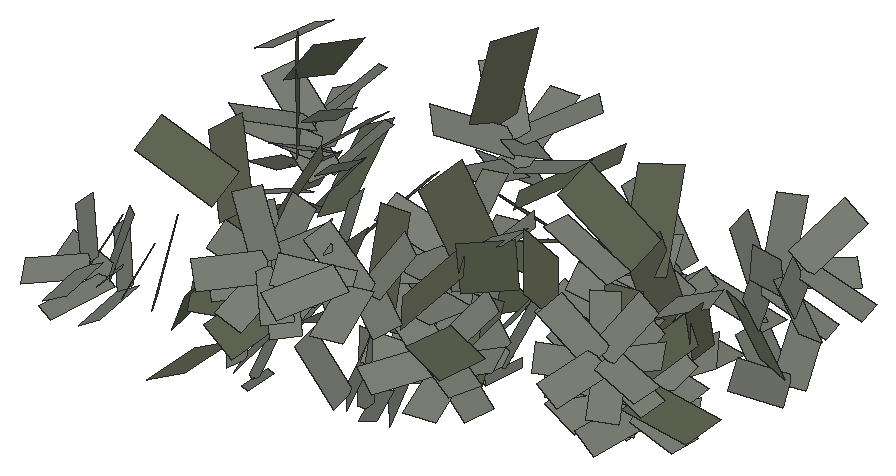
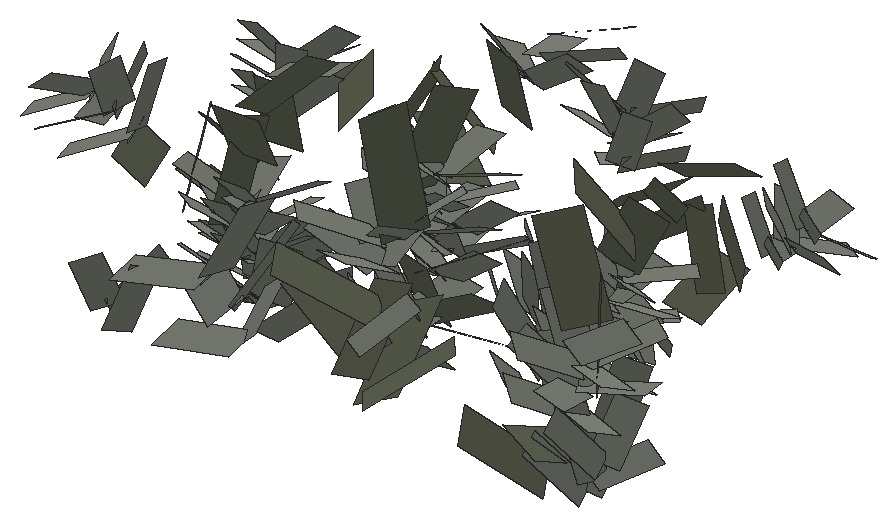
# SketchUp Ruby script. Lengths in inches.
U = 1.inch
M = Sketchup.active_model
def pt(a) = Geom::Point3d.new(a.map { |v| v * U })
def face(e, loops, mat)
  f = e.add_face(loops[0].map { |a| pt(a) })
  loops[1..].each { |l| e.add_face(l.map { |a| pt(a) }).erase! }
  f.material = f.back_material = mat if mat
  f
end
# faces: each face lists its corners as indices into pts; further lists are holes
def faces(e, pts, list, mat = nil) = list.each { |f| face(e, (f[0].is_a?(Array) ? f : [f]).map { |l| l.map { |i| pts[i] } }, mat) }
# xy, xz, yz: faces in a plane at the given z, y or x. An outline is a flat list of corners, or four numbers for a rectangle; further outlines are holes
def ring(l) = l.size == 4 ? [[l[0], l[1]], [l[2], l[1]], [l[2], l[3]], [l[0], l[3]]] : l.each_slice(2).to_a
def flat(e, list, mat, &to3) = list.each { |f| face(e, (f[0].is_a?(Array) ? f : [f]).map { |l| ring(l).map { |u, v| to3.(u, v) } }, mat) }
def xy(e, z, list, mat = nil) = flat(e, list, mat) { |x, y| [x, y, z] }
def xz(e, y, list, mat = nil) = flat(e, list, mat) { |x, z| [x, y, z] }
def yz(e, x, list, mat = nil) = flat(e, list, mat) { |y, z| [x, y, z] }
def lines(e, pts, list) = list.each { |a, b| e.add_line(pt(pts[a]), pt(pts[b])) }
# prism: a flat outline (further loops are holes) pulled along v
def prism(e, loops, v, mat = nil)
  f = face(e, loops, mat); d = Geom::Vector3d.new(v.map { |x| x * U })
  f.pushpull(f.normal.samedirection?(d) ? d.length : -d.length)
end
def box(e, o, s, mat = nil) = prism(e, [[o, [o[0] + s[0], o[1], o[2]], [o[0] + s[0], o[1] + s[1], o[2]], [o[0], o[1] + s[1], o[2]]]], [0, 0, s[2]], mat)
def at(x, y, z, deg = 0) = Geom::Transformation.translation(pt([x, y, z])) * Geom::Transformation.rotation(ORIGIN, Z_AXIS, deg.degrees)
def axes(o, x, y, z) = Geom::Transformation.new([*x, 0, *y, 0, *z, 0, *pt(o).to_a, 1])
def part(name) = M.definitions.add(name)
# library, detail: a bought-in or finely detailed component or shape, given as its bounding box
def library(name, o, s) = part(name).tap { |d| box(d.entities, o, s) }
def detail(e, o, s) = box(e.add_group.entities, o, s)
def put(e, d, t, mat = nil) = e.add_instance(d, t).tap { |i| i.material = mat if mat }
def group(e, t, mat = nil) = e.add_group.tap { |g| g.transformation = t; g.material = mat if mat }.entities
root = M.entities
M.materials.add("viburnumblaasdfas0df1w06d").color = [98, 102, 84]
M.materials.add("viburnumbladsadfasdfad0w122").color = [125, 129, 119]
c1 = part("Component\#315")
p = [[0.25,0,0],[2.05,0.01,0.35],[1.81,4.2,1.66],[0,4.19,1.3125]]
faces(c1.entities,p,[[0,1,2,3]],"viburnumbladsadfasdfad0w122")
c2 = part("viburnumblad2")
put(c2.entities,c1,axes([-19.23,-4.49,-32.18],[83.35428,0,0],[0,79.38502,0],[0,0,83.35428]))
c3 = part("Component\#314")
p = [[0.14,0,0],[2.58,0.05,0.25],[2.44,5.11,2.64],[0,5.05,2.39]]
faces(c3.entities,p,[[0,1,2,3]],"viburnumblaasdfas0df1w06d")
c4 = part("viburnumblad1\#2")
put(c4.entities,c3,axes([-37.25,6.23,19.31],[75.98784,0,0],[0,65.50676,0],[0,0,75.98784]))
put(root,c2,axes([2210.98,245.61,41],[-0.00995,0.00489,0.00397],[-0.00628,-0.00876,-0.0047],[0.00102,-0.00608,0.00892]))
put(root,c2,axes([2194.08,246.49,36.46],[-0.00855,-0.00051,-0.00592],[0.00282,-0.00961,-0.00317],[-0.00532,-0.00402,0.00702]))
put(root,c2,axes([2211.35,247.21,40.45],[-0.01153,-0.00217,-0.00126],[0.00257,-0.00998,-0.00587],[-0.00007,-0.00594,0.00905]))
put(root,c2,axes([2194.73,246.58,35.24],[-0.00848,0.00604,-0.00136],[-0.00422,-0.00741,-0.00622],[-0.00446,-0.0043,0.00739]))
put(root,c2,axes([2204.71,247.03,38.64],[-0.00593,0.00534,0.00783],[-0.0086,-0.00691,-0.00181],[0.00397,-0.00698,0.00778]))
put(root,c2,axes([2193.45,245.78,35.56],[-0.00345,0.00905,0.004],[-0.00908,-0.00113,-0.00507],[-0.00385,-0.00506,0.00725]))
put(root,c2,axes([2195.31,247.78,34.96],[-0.00729,-0.00007,-0.00611],[0.00282,-0.00961,-0.00317],[-0.00621,-0.00405,0.00634]))
put(root,c2,axes([2210.35,246.29,39.8],[-0.00254,0.00908,0.00688],[-0.01141,-0.00302,-0.00024],[0.00165,-0.00679,0.00837]))
put(root,c2,axes([2194.26,247.87,35.79],[-0.0036,-0.00676,-0.00701],[0.00718,-0.00608,0.00197],[-0.00593,-0.00439,0.00637]))
put(root,c2,axes([2205.21,248.04,39.49],[-0.00902,-0.00601,-0.00274],[0.00624,-0.00625,-0.00686],[0.00215,-0.00706,0.0084]))
put(root,c2,axes([2193.1,247.39,36.44],[0.00345,-0.00905,-0.004],[0.00788,-0.00012,0.00668],[-0.00594,-0.00519,0.00581]))
put(root,c2,axes([2204.74,248.61,38.12],[-0.01058,-0.00047,0.0036],[-0.00191,-0.00936,-0.00683],[0.00314,-0.00674,0.00835]))
put(root,c2,axes([2210.85,248.58,39.97],[-0.00572,-0.00664,-0.00612],[0.0099,-0.00571,-0.00294],[-0.00165,-0.00728,0.00803]))
put(root,c2,axes([2194.49,248.56,34.85],[0.0036,-0.00945,-0.00418],[0.00709,-0.00011,0.00601],[-0.00594,-0.00519,0.00581]))
put(root,c2,axes([2193.57,246.69,34.57],[0.0036,0.00676,0.00701],[-0.00902,0.00536,-0.00055],[-0.00386,-0.00586,0.0067]))
put(root,c2,axes([2192.47,246.68,35.54],[0.00855,0.00051,0.00592],[-0.00403,0.00835,0.00477],[-0.00448,-0.00623,0.00604]))
put(root,c2,axes([2203.74,247.87,37.72],[0.00218,0.00802,0.00747],[-0.00931,-0.0013,0.00412],[0.00416,-0.00766,0.007]))
put(root,c2,axes([2203.44,247.14,39.25],[0.00902,0.00601,0.00274],[-0.00554,0.00435,0.00868],[0.0036,-0.00837,0.00649]))
put(root,c2,axes([2203.78,248.93,36.85],[-0.0062,0.00558,0.00817],[-0.00774,-0.00622,-0.00163],[0.00397,-0.00698,0.00778]))
put(root,c2,axes([2193.28,247.72,35.06],[0.00848,-0.00604,0.00136],[0.00312,0.00638,0.00815],[-0.00533,-0.00595,0.00568]))
put(root,c2,axes([2204.16,249.98,37.74],[-0.00866,-0.00577,-0.00263],[0.00674,-0.00675,-0.0074],[0.00215,-0.00706,0.0084]))
put(root,c4,axes([2199,251.1875,31.14],[-0.01085,-0.00246,-0.00558],[0.00478,-0.01321,-0.00344],[-0.00438,-0.00417,0.00964]))
put(root,c2,axes([2209.78,247.375,38.95],[0.00611,0.00764,0.00552],[-0.01063,0.0043,0.00535],[0.00146,-0.00765,0.00773]))
put(root,c2,axes([2203.94,248.15,40.1],[0.00593,-0.00534,-0.00783],[0.00931,0.00502,0.00364],[0.00177,-0.00845,0.00711]))
put(root,c4,axes([2203.52,251.18,35.08],[-0.00973,0.00003,0.00746],[-0.00524,-0.01136,-0.00678],[0.00594,-0.00739,0.00778]))
put(root,c2,axes([2204.17,249.26,39.05],[-0.00218,-0.00802,-0.00747],[0.01085,-0.00048,-0.00266],[0.00158,-0.00777,0.00788]))
put(root,c2,axes([2209.59,248.52,39.87],[0.01038,-0.0051,-0.00415],[0.00571,0.00633,0.00604],[-0.00053,-0.00802,0.00751]))
put(root,c2,axes([2193.96,247.78,33.93],[0.00821,0.00049,0.00568],[-0.00435,0.00902,0.00515],[-0.00448,-0.00623,0.00604]))
put(root,c4,axes([2196.98,251,32.46],[-0.00104,-0.01037,-0.00489],[0.01073,-0.00422,0.00645],[-0.0067,-0.00317,0.00766]))
put(root,c2,axes([2202.91,248.6,38.84],[0.01058,0.00047,-0.0036],[0.00255,0.00709,0.00842],[0.00261,-0.00869,0.00653]))
put(root,c4,axes([2195.3,249.85,32.91],[0.00672,-0.00928,0.00091],[0.00601,0.00561,0.01016],[-0.00772,-0.00461,0.00599]))
put(root,c2,axes([2202.7,248.93,37.39],[0.0079,0.00633,0.00186],[-0.00554,0.00435,0.00868],[0.00455,-0.00767,0.00675]))
put(root,c4,axes([2202.2,251.8,33.3125],[-0.0017,0.006,0.01056],[-0.01273,-0.00619,0.00147],[0.00521,-0.00927,0.00611]))
put(root,c2,axes([2223.12,252.09,37.56],[-0.00968,0.00131,0.00494],[-0.00342,-0.0096,-0.00398],[0.00374,-0.00505,0.00789]))
put(root,c4,axes([2209.18,249.93,37.5],[0.01273,-0.00184,0.00122],[0.00029,0.0105,0.01027],[-0.0024,-0.00896,0.00784]))
put(root,c4,axes([2211.03,253.68,35.06],[-0.00662,-0.01127,-0.00498],[0.01432,-0.00702,-0.0031],[-0.00011,-0.00548,0.01154]))
put(root,c4,axes([2198.26,251.09,39.05],[0.0023,0.0101,0.00657],[-0.0138,0.00343,-0.00044],[-0.0019,-0.0063,0.01035]))
put(root,c2,axes([2199.6,253.16,29.28],[-0.00404,-0.00727,-0.00631],[0.00772,-0.00559,0.00142],[-0.00472,-0.00433,0.00722]))
put(root,c2,axes([2222.91,253.6,37.07],[-0.00956,-0.00538,0.00002],[0.00454,-0.00801,-0.00608],[0.00277,-0.00525,0.00814]))
put(root,c4,axes([2209.58,252.1,36.74],[0.00746,-0.00961,-0.00443],[0.01187,0.00604,0.00656],[-0.00274,-0.0068,0.00947]))
put(root,c2,axes([2222.24,252.5,36.54],[-0.00413,0.00723,0.00696],[-0.00909,-0.00609,0.00092],[0.00444,-0.00548,0.00729]))
put(root,c2,axes([2211.08,253.23,32.95],[-0.00995,0.00489,0.00397],[-0.00607,-0.00954,-0.00338],[0.0019,-0.00477,0.00949]))
put(root,c2,axes([2222.8125,253.1,38.42],[-0.00385,-0.00891,-0.00491],[0.01001,-0.00205,-0.00401],[0.00209,-0.00597,0.00789]))
put(root,c2,axes([2198.58,252.66,30.09],[0.00345,-0.00905,-0.004],[0.00865,0.00062,0.00578],[-0.00475,-0.00515,0.0067]))
put(root,c2,axes([2221.84,251.57,37.71],[0.00385,0.00891,0.00491],[-0.00921,0.00054,0.0058],[0.00445,-0.00629,0.00669]))
put(root,c2,axes([2205.17,252.5,30.47],[0.00814,-0.00715,-0.0046],[0.00716,0.00216,0.00888],[-0.00455,-0.00881,0.00477]))
put(root,c2,axes([2206.23,253.59,30.01],[0.00034,-0.00733,-0.00907],[0.00978,-0.00348,0.00299],[-0.00497,-0.00808,0.00546]))
put(root,c2,axes([2201.07,254.11,33.14],[-0.0105,0.00104,-0.00371],[-0.00071,-0.0111,-0.00111],[-0.00379,-0.00081,0.01049]))
put(root,c2,axes([2200.22,253.1,34.15],[-0.00725,0.00846,-0.00094],[-0.008,-0.0072,-0.00303],[-0.00289,-0.00129,0.01072]))
put(root,c2,axes([2204.97,251.64,29.28],[0.00766,0.00322,0.00823],[-0.00853,0.00606,0.00527],[-0.00262,-0.00929,0.00521]))
put(root,c2,axes([2200.47,254.44,34.53],[-0.00759,-0.00699,-0.00431],[0.00673,-0.00866,0.00218],[-0.0047,-0.00111,0.01008]))
put(root,c2,axes([2211.33,254.75,32.21],[-0.01146,-0.00283,-0.00038],[0.00275,-0.01049,-0.00491],[0.00082,-0.00467,0.00968]))
put(root,c2,axes([2211,254.51,33.7],[-0.00626,-0.00889,-0.00451],[0.01001,-0.00557,-0.00285],[-0.00007,-0.00526,0.00943]))
put(root,c2,axes([2197.88,251.875,29.29],[0.00916,0.00124,0.00492],[-0.00387,0.00837,0.00487],[-0.00322,-0.0061,0.00681]))
put(root,c2,axes([2201.2,253.98,31.65],[-0.00696,0.00812,-0.0009],[-0.00864,-0.00777,-0.00327],[-0.00289,-0.00129,0.01072]))
put(root,c4,axes([2200.31,253.49,32.35],[0.01074,0.00549,0.00552],[-0.0086,0.00502,0.01173],[0.00238,-0.01127,0.00657]))
put(root,c2,axes([2198.55,252.93,28.67],[0.00892,-0.00552,0.00065],[0.00374,0.00694,0.00752],[-0.00413,-0.00589,0.00653]))
put(root,c2,axes([2221.53,252.59,38.57],[0.00968,-0.00131,-0.00494],[0.00422,0.00809,0.00577],[0.0028,-0.00722,0.00669]))
put(root,c2,axes([2222.01,254.66,36.73],[-0.00372,-0.00756,-0.00527],[0.01001,-0.00205,-0.00401],[0.00166,-0.0069,0.00731]))
put(root,c2,axes([2210.34,253.72,31.72],[-0.00261,0.00974,0.006],[-0.01123,-0.00353,0.00072],[0.00254,-0.00551,0.00899]))
put(root,c2,axes([2205.4,253.14,29.01],[0.01118,-0.00278,0.00257],[-0.00082,0.00655,0.0102],[-0.00357,-0.00931,0.00467]))
put(root,c2,axes([2221.32,253.28,35.86],[0.00369,0.00856,0.00471],[-0.00994,0.00059,0.00626],[0.00445,-0.00629,0.00669]))
put(root,c2,axes([2221.53,253.81,37.75],[0.00413,-0.00723,-0.00696],[0.00908,0.00421,0.0008],[0.0021,-0.00679,0.00729]))
put(root,c4,axes([2197.78,252.36,37.22],[0.01004,0.00303,0.00636],[-0.00636,0.01197,0.00433],[-0.00443,-0.0059,0.0098]))
put(root,c2,axes([2221.18,252.74,37.13],[0.00956,0.00538,-0.00002],[-0.00388,0.00674,0.0082],[0.00377,-0.00701,0.00644]))
put(root,c2,axes([2206.29,254.55,29.09],[0.0085,-0.00746,-0.0048],[0.00645,0.00195,0.00799],[-0.00455,-0.00881,0.00477]))
put(root,c2,axes([2209.59,253.09,33.03],[0.00626,0.00889,0.00451],[-0.00973,0.00413,0.00504],[0.00235,-0.00645,0.00846]))
put(root,c2,axes([2200.15,253.41,32.62],[0.00024,0.01092,0.00238],[-0.01143,0.00081,-0.00255],[-0.00254,-0.00227,0.01065]))
put(root,c2,axes([2200.3,255.32,33.1],[-0.00024,-0.01092,-0.00238],[0.01005,-0.00131,0.00499],[-0.0051,-0.00202,0.00975]))
put(root,c2,axes([2210.73,256.02,31.61],[-0.00572,-0.00761,-0.00506],[0.01001,-0.00557,-0.00285],[-0.00075,-0.00619,0.00889]))
put(root,c4,axes([2213.08,256.98,37.12],[-0.00612,0.00474,0.0114],[-0.00511,-0.01476,0.0034],[0.01154,-0.00234,0.00716]))
put(root,c2,axes([2210.47,256.54,38.125],[-0.01249,0.00076,-0.00112],[-0.00058,-0.01239,-0.00197],[-0.00123,-0.0019,0.01236]))
put(root,c2,axes([2209.92,255.46,32.74],[0.00261,-0.00974,-0.006],[0.01057,0.00192,0.00135],[-0.00026,-0.0062,0.0089]))
put(root,c4,axes([2214.61,257.77,39.02],[-0.00769,-0.00672,0.00925],[0.00492,-0.01396,-0.00605],[0.01062,-0.00006,0.00878]))
put(root,c2,axes([2220.91,254.23,36.77],[0.01011,-0.00136,-0.00516],[0.0038,0.00729,0.00519],[0.0028,-0.00722,0.00669]))
put(root,c2,axes([2209.52,254.36,33.79],[0.00995,-0.00489,-0.00397],[0.00635,0.0081,0.00558],[0.00038,-0.00694,0.0084]))
put(root,c4,axes([2198.54,254.38,35.57],[0.00884,-0.00966,0.00214],[0.00883,0.00982,0.0079],[-0.00632,-0.00331,0.01118]))
put(root,c2,axes([2198.92,253.47,33.74],[0.00759,0.00699,0.00431],[-0.00767,0.00813,0.00032],[-0.00293,-0.00317,0.01031]))
put(root,c2,axes([2200.8125,257.29,32.66],[-0.0119,0.00385,-0.00772],[-0.00199,-0.01402,-0.00394],[-0.0084,-0.00214,0.01187]))
put(root,c2,axes([2199.17,254.8,34.11],[0.00725,-0.00846,0.00094],[0.00707,0.00667,0.00553],[-0.00474,-0.00299,0.00967]))
put(root,c2,axes([2210.54,257.68,35.17],[-0.01199,0.00073,-0.00108],[-0.00063,-0.01339,-0.00213],[-0.00123,-0.0019,0.01236]))
put(root,c2,axes([2210.17,256.53,36.4],[-0.00853,0.00907,0.00165],[-0.00968,-0.00877,-0.00184],[-0.00017,-0.0024,0.01233]))
put(root,c2,axes([2209.66,254.64,30.78],[0.00601,0.00853,0.00433],[-0.01051,0.00446,0.00545],[0.00235,-0.00645,0.00846]))
put(root,c2,axes([2199.24,254.34,32.46],[0.0105,-0.00104,0.00371],[-0.00021,0.00971,0.00332],[-0.00385,-0.00347,0.00991]))
put(root,c2,axes([2210.34,257.88,36.82],[-0.00913,-0.008,-0.00324],[0.00831,-0.00942,-0.00017],[-0.00232,-0.00227,0.01214]))
put(root,c2,axes([2199.86,254.22,31.24],[0.00793,0.00729,0.0045],[-0.0069,0.00732,0.00029],[-0.00293,-0.00317,0.01031]))
put(root,c2,axes([2199.99,255.36,31.625],[0.0071,-0.00744,-0.0001],[0.00707,0.00667,0.00553],[-0.00393,-0.00389,0.00972]))
put(root,c2,axes([2209.28,254.36,32.1875],[0.01146,0.00283,0.00038],[-0.00257,0.0094,0.00741],[0.00146,-0.00704,0.00821]))
put(root,c4,axes([2219.86,255.35,34.68],[0.0118,0.00221,-0.00034],[-0.00169,0.00933,0.00984],[0.00149,-0.00861,0.00716]))
put(root,c4,axes([2210.24,257.55,31.83],[-0.0066,0.01089,0.00527],[-0.0139,-0.00777,-0.00135],[0.00164,-0.00514,0.01268]))
put(root,c2,axes([2201.65,258.88,31.42],[-0.00909,-0.00693,-0.00924],[0.00664,-0.01276,0.00304],[-0.00946,-0.0023,0.01102]))
put(root,c2,axes([2209.15,255.74,37.76],[0.00042,0.01207,0.00346],[-0.01255,0.00034,0.00035],[0.00024,-0.00347,0.01207]))
put(root,c2,axes([2209.46,255.89,31.57],[0.01038,-0.0051,-0.00415],[0.00572,0.00729,0.00502],[0.00038,-0.00694,0.0084]))
put(root,c4,axes([2210.23,256.6875,36.08],[0.00411,0.01355,0.00465],[-0.01078,-0.00135,0.01345],[0.01091,-0.00609,0.00813]))
put(root,c2,axes([2216.09,257.6875,42.04],[-0.00224,-0.01174,-0.0016],[0.0107,-0.00091,-0.00829],[0.00736,-0.00274,0.0098]))
put(root,c2,axes([2209.61,257.84,38.4],[-0.00042,-0.01207,-0.00346],[0.01224,-0.00117,0.00258],[-0.0028,-0.00328,0.0118]))
put(root,c2,axes([2209.79,259.3,31.41],[-0.01244,-0.00019,-0.00567],[0.00199,-0.01294,-0.00394],[-0.00531,-0.00441,0.0118]))
put(root,c2,axes([2220,258.82,30.4],[-0.00968,0.00131,0.00494],[-0.00285,-0.01022,-0.00281],[0.00419,-0.00363,0.00837]))
put(root,c2,axes([2200.04,258.98,32.65],[-0.00095,-0.01366,-0.00535],[0.01077,-0.00429,0.00904],[-0.00996,-0.00334,0.01028]))
put(root,c2,axes([2209.29,256.75,34.8125],[0.00044,0.0126,0.00361],[-0.0113,0.00031,0.00032],[0.00024,-0.00347,0.01207]))
put(root,c4,axes([2220.07,259.2,32.36],[-0.00299,-0.01191,-0.00429],[0.01424,-0.00187,-0.0047],[0.00288,-0.00486,0.01046]))
put(root,c4,axes([2219.47,257.38,34.02],[0.00886,-0.00621,-0.00526],[0.00932,0.00889,0.00498],[0.00073,-0.00681,0.00878]))
put(root,c4,axes([2208.83,256.94,29.08],[0.01287,-0.00107,0.00071],[0.00034,0.01171,0.00907],[-0.00141,-0.0079,0.00892]))
put(root,c2,axes([2199.51,256.69,31.47],[0.00095,0.01366,0.00535],[-0.01286,0.00336,-0.00628],[-0.00706,-0.00428,0.01216]))
put(root,c2,axes([2208.7,256.52,36.22],[0.00913,0.008,0.00324],[-0.00792,0.00789,0.00285],[-0.00024,-0.00448,0.01173]))
put(root,c2,axes([2219.07,259.03,29.36],[-0.00449,0.00779,0.00619],[-0.00867,-0.00648,0.00177],[0.0049,-0.00408,0.00781]))
put(root,c2,axes([2218.16,260.82,31.47],[-0.01366,0.00095,0.00535],[-0.00336,-0.01286,-0.00628],[0.00428,-0.00706,0.01216]))
put(root,c2,axes([2208.76,258.21,36.74],[0.00853,-0.00907,-0.00165],[0.009,0.0076,0.00473],[-0.00239,-0.00435,0.01154]))
put(root,c2,axes([2208.29,257.04,38.03],[0.01249,-0.00076,0.00112],[0.00026,0.01157,0.0049],[-0.00133,-0.00485,0.01151]))
put(root,c2,axes([2209.91,260.96,30.23],[-0.00694,-0.00883,-0.00779],[0.00996,-0.00923,0.0016],[-0.00629,-0.00487,0.01112]))
put(root,c4,axes([2209.16,257.96,29.54],[0.0051,0.011,0.00655],[-0.01483,0.00551,0.0023],[-0.00067,-0.00681,0.01196]))
put(root,c2,axes([2219.64,259.92,31.15],[-0.00334,-0.0097,-0.00381],[0.01007,-0.00189,-0.00393],[0.0026,-0.00465,0.00851]))
put(root,c2,axes([2218.76,258.25,30.63],[0.00334,0.0097,0.00381],[-0.00915,0.00071,0.00588],[0.00496,-0.00497,0.00731]))
put(root,c2,axes([2208.7,258.39,30.4375],[-0.00263,0.0123,0.00535],[-0.01296,-0.00091,-0.00426],[-0.00348,-0.00589,0.01184]))
put(root,c4,axes([2218.99,259.29,38.87],[0.00217,0.0115,0.00524],[-0.01369,-0.00006,0.0058],[0.00451,-0.00566,0.01058]))
put(root,c2,axes([2208.62,260.56,31.55],[0.00263,-0.0123,-0.00535],[0.01173,-0.00054,0.007],[-0.00651,-0.00594,0.01045]))
put(root,c2,axes([2219.08,261.55,35.37],[-0.01126,-0.00309,0.00036],[0.00297,-0.01108,-0.00222],[0.00093,-0.00205,0.01147]))
put(root,c2,axes([2208.49,257.8,35.125],[0.01156,-0.00022,-0.00012],[0.00026,0.01157,0.0049],[0.00003,-0.0049,0.01157]))
put(root,c2,axes([2195.63,261.61,29.54],[-0.00877,-0.00751,-0.00615],[0.00336,-0.01013,0.00757],[-0.0091,0.00349,0.00872]))
put(root,c2,axes([2200.17,259.63,30.53],[0.00774,-0.01238,0.00167],[0.00805,0.00648,0.01066],[-0.00962,-0.00465,0.01009]))
put(root,c2,axes([2200.05,257.71,29.75],[0.00909,0.00693,0.00924],[-0.00802,0.01085,-0.00026],[-0.00757,-0.00532,0.01142]))
put(root,c2,axes([2218.625,261.46,33.81],[-0.00997,0.00542,0.0028],[-0.00605,-0.01063,-0.00096],[0.002,-0.00216,0.01131]))
put(root,c2,axes([2198.75,258.38,31.47],[0.0119,-0.00385,0.00772],[-0.0001,0.01309,0.00669],[-0.00863,-0.00547,0.01057]))
put(root,c2,axes([2218.09,259.64,28.61],[0.0032,0.00932,0.00366],[-0.00988,0.00076,0.00635],[0.00496,-0.00497,0.00731]))
put(root,c2,axes([2218.46,262.58,32.67],[-0.01081,-0.00296,0.00035],[0.0032,-0.01197,-0.0024],[0.00093,-0.00205,0.01147]))
put(root,c2,axes([2217.14,261.36,29.75],[-0.00693,0.00909,0.00924],[-0.01085,-0.00802,-0.00026],[0.00532,-0.00757,0.01142]))
put(root,c4,axes([2217.85,262.37,29.62],[-0.0084,0.0076,0.00599],[-0.00998,-0.01102,-0.00002],[0.00443,-0.00403,0.01133]))
put(root,c2,axes([2218.13,260.45,35.14],[-0.00283,0.01075,0.0036],[-0.01102,-0.00348,0.00171],[0.00265,-0.00298,0.01098]))
put(root,c2,axes([2218.31,260.43,30.42],[0.00449,-0.00779,-0.00619],[0.00881,0.00487,0.00016],[0.00266,-0.00553,0.00801]))
put(root,c2,axes([2218.4,259.35,31.39],[0.00968,-0.00131,-0.00494],[0.00378,0.00904,0.00475],[0.00337,-0.00599,0.00744]))
put(root,c2,axes([2216.47,260.05,31.47],[0.00385,0.0119,0.00772],[-0.01309,-0.0001,0.00669],[0.00547,-0.00863,0.01057]))
put(root,c4,axes([2221.12,262.73,34.17],[-0.00543,0.00233,0.01137],[0.00034,-0.01453,0.00314],[0.0116,0.00141,0.00526]))
put(root,c2,axes([2218.01,259.28,29.9375],[0.0092,0.00594,-0.0008],[-0.00419,0.00749,0.00747],[0.00433,-0.00576,0.00715]))
put(root,c2,axes([2217.5625,262.12,32.66],[-0.00385,-0.0119,-0.00772],[0.01402,-0.00199,-0.00394],[0.00214,-0.0084,0.01187]))
put(root,c2,axes([2208.67,259.45,28.82],[0.00694,0.00883,0.00779],[-0.01027,0.00714,0.00105],[-0.0037,-0.00696,0.01117]))
put(root,c2,axes([2200.69,259.26,28.67],[0.01174,-0.00298,0.00601],[-0.0001,0.01309,0.00669],[-0.00729,-0.00586,0.01134]))
put(root,c2,axes([2218.42,262.6875,34.23],[-0.00596,-0.00978,-0.00229],[0.01005,-0.00579,-0.00143],[0.00006,-0.0027,0.01137]))
put(root,c2,axes([2207.53,259.64,30.58],[0.01244,0.00019,0.00567],[-0.00322,0.01148,0.00668],[-0.00467,-0.00741,0.01049]))
put(root,c4,axes([2218.59,261.61,33.51],[0.00008,0.01316,0.00435],[-0.00745,-0.00443,0.01354],[0.01228,-0.00208,0.00607]))
put(root,c2,axes([2217.6,261.38,32.45],[-0.00295,0.01122,0.00376],[-0.00992,-0.00313,0.00154],[0.00265,-0.00298,0.01098]))
put(root,c2,axes([2224.84,263.32,37.51],[-0.00724,-0.00234,0.00954],[0.00229,-0.01023,-0.00078],[0.00905,0.00148,0.00724]))
put(root,c2,axes([2227.21,263.54,39.16],[-0.00693,-0.00224,0.00913],[0.00254,-0.01137,-0.00086],[0.00905,0.00148,0.00724]))
put(root,c2,axes([2208.29,261.17,29.61],[0.01065,-0.00857,0.00023],[0.00633,0.00812,0.0092],[-0.00584,-0.00699,0.01019]))
put(root,c2,axes([2217.64,260.67,29.41],[0.01011,-0.00136,-0.00516],[0.0034,0.00814,0.00428],[0.00337,-0.00599,0.00744]))
put(root,c4,axes([2222.4375,263.88,35.79],[-0.00364,-0.00823,0.00913],[0.00776,-0.0108,-0.00665],[0.01031,0.00314,0.00694]))
put(root,c2,axes([2225.9,262.9,38.375],[-0.00591,0.00652,0.00769],[-0.00251,-0.00882,0.00556],[0.0097,0.00126,0.00639]))
put(root,c2,axes([2217.97,262.4375,35.76],[0.00283,-0.01075,-0.0036],[0.01134,0.00265,0.001],[-0.0001,-0.00373,0.01107]))
put(root,c2,axes([2217.33,261,33.8],[0.00596,0.00978,0.00229],[-0.00894,0.00456,0.00379],[0.00249,-0.00402,0.01069]))
put(root,c2,axes([2215.59,262,28.67],[0.00298,0.01174,0.00601],[-0.01309,-0.0001,0.00669],[0.00586,-0.00729,0.01134]))
put(root,c2,axes([2225.68,264.23,38.67],[-0.0039,-0.00969,0.00523],[0.00734,-0.00679,-0.00711],[0.00851,0.00087,0.00796]))
put(root,c4,axes([2217.27,260.72,37.12],[0.01321,0.00417,0.00061],[-0.00463,0.0136,0.00723],[0.00136,-0.00611,0.01237]))
put(root,c2,axes([2215.875,261.35,32.65],[0.01366,-0.00095,-0.00535],[0.00429,0.01077,0.00904],[0.00334,-0.00996,0.01028]))
put(root,c2,axes([2224.42,262.37,38.22],[-0.0023,0.01045,0.001],[-0.00575,-0.00222,0.00993],[0.00986,0.00159,0.00606]))
put(root,c2,axes([2215.22,261.47,30.53],[0.01238,0.00774,0.00167],[-0.00648,0.00805,0.01066],[0.00465,-0.00962,0.01009]))
put(root,c2,axes([2217.02,261.34,35.54],[0.01126,0.00309,-0.00036],[-0.00265,0.01026,0.00493],[0.00162,-0.00467,0.01059]))
put(root,c2,axes([2215.97,262.96,31.42],[0.00693,-0.00909,-0.00924],[0.01276,0.00664,0.00304],[0.0023,-0.00946,0.01102]))
put(root,c2,axes([2194.78,265.26,35.14],[-0.01197,-0.00238,-0.00293],[0.00194,-0.01232,0.00219],[-0.00304,0.00182,0.01144]))
put(root,c2,axes([2193.98,264.39,36.52],[-0.01008,0.00703,-0.00261],[-0.00714,-0.01028,-0.00011],[-0.00193,0.00159,0.01172]))
put(root,c4,axes([2206.62,266.62,29.26],[-0.01489,-0.00148,0.00524],[0.00198,-0.01828,0.00047],[0.00517,0.00094,0.01496]))
put(root,c2,axes([2207,265.66,37.82],[-0.01229,-0.00021,0.00042],[0.00023,-0.01336,0.00026],[0.00045,0.00027,0.01335]))
put(root,c2,axes([2216.93,262.5,34.34],[0.00997,-0.00542,-0.0028],[0.00614,0.00939,0.00366],[0.00055,-0.00455,0.01075]))
put(root,c2,axes([2206.8,264.61,39.26],[-0.00935,0.00927,0.0023],[-0.00914,-0.00973,0.00201],[0.00303,-0.00016,0.01302]))
put(root,c2,axes([2216.63,262.0625,32.86],[0.01014,0.00329,-0.00138],[-0.00265,0.01026,0.00493],[0.00283,-0.00431,0.01049]))
put(root,c2,axes([2224.1,264.25,38.4],[0.00136,-0.01101,-0.00167],[0.00866,0.00241,-0.00886],[0.00838,-0.00019,0.00814]))
put(root,c4,axes([2193.41,266.07,38.15],[-0.00759,-0.01277,-0.00082],[0.01374,-0.0085,0.0061],[-0.0047,0.00228,0.01321]))
put(root,c2,axes([2226.56,264.5625,40],[0.00142,-0.01147,-0.00174],[0.00801,0.00224,-0.0082],[0.00838,-0.00019,0.00814]))
put(root,c2,axes([2193.96,265.97,36.49],[-0.00685,-0.0104,-0.00154],[0.00967,-0.00694,0.00401],[-0.00399,0.00118,0.01121]))
put(root,c2,axes([2194.63,266.02,33.71],[-0.00587,-0.00963,-0.00252],[0.00967,-0.00694,0.00401],[-0.00471,0.00005,0.01098]))
put(root,c2,axes([2224.95,262.59,39.68],[0.0039,0.00969,-0.00523],[-0.00478,0.00655,0.00858],[0.00995,-0.00072,0.00609]))
put(root,c2,axes([2206.8,266.49,39.42],[-0.00935,-0.00954,0.00039],[0.00874,-0.00859,-0.00062],[0.00075,-0.0002,0.01334]))
put(root,c2,axes([2217.18,266.92,33.6],[-0.01234,0.00028,0.00961],[0.00075,-0.01555,0.00142],[0.00958,0.00158,0.01226]))
put(root,c4,axes([2192.77,264.91,34.28],[0.0095,-0.01111,0.00288],[0.00361,0.00703,0.01484],[-0.01096,-0.00785,0.00554]))
put(root,c2,axes([2193.72,264.07,34.9],[-0.00228,0.01232,-0.00076],[-0.01222,-0.00233,-0.0015],[-0.0013,0.00061,0.01189]))
put(root,c2,axes([2214.99,267.08,30.57],[-0.01223,0.0001,0.00757],[0.00075,-0.01555,0.00142],[0.00819,0.0016,0.01322]))
put(root,c2,axes([2215.65,266,32.24],[-0.00842,0.01125,0.00685],[-0.00786,-0.01092,0.00827],[0.01063,0.001,0.01143]))
put(root,c2,axes([2192.64,266.87,30.28],[-0.00935,-0.0054,-0.00582],[0.00328,-0.00946,0.00316],[-0.00651,0.0014,0.00804]))
put(root,c4,axes([2205.18,266.3125,39.27],[-0.00382,-0.01538,-0.00062],[0.0121,-0.00355,0.01339],[-0.01131,0.00237,0.01086]))
put(root,c2,axes([2191.99,266.45,31.29],[-0.00946,0.00383,-0.00571],[-0.0036,-0.01015,-0.00104],[-0.00558,0.00147,0.00861]))
put(root,c2,axes([2191.2,267.12,32.39],[-0.00896,-0.00518,-0.00557],[0.00365,-0.01051,0.00351],[-0.00651,0.0014,0.00804]))
put(root,c2,axes([2224.91,264.09,39.73],[0.00591,-0.00652,-0.00769],[0.005,0.00963,-0.00433],[0.00875,-0.0011,0.00766]))
put(root,c2,axes([2223.21,266.28,29.28],[-0.00322,0.00766,0.00823],[-0.00606,-0.00853,0.00527],[0.00929,-0.00262,0.00521]))
put(root,c2,axes([2225.94,263.5,40.82],[0.00693,0.00224,-0.00913],[-0.00028,0.01139,0.00259],[0.0094,-0.00132,0.00681]))
put(root,c2,axes([2193.37,266.25,34.74],[0.00228,-0.01232,0.00076],[0.0106,0.00221,0.00397],[-0.00422,0.00003,0.01117]))
put(root,c2,axes([2206.11,266.78,37.96],[0,-0.01388,-0.00141],[0.01203,0.00003,-0.00025],[0.00028,-0.00135,0.01329]))
put(root,c2,axes([2215.68,268.21,32.22],[-0.00902,-0.01086,0.00673],[0.00875,-0.01029,-0.00487],[0.0085,0.00104,0.01308]))
put(root,c4,axes([2206.01,267.69,32.27],[-0.00484,-0.01365,0.00231],[0.016,-0.00575,-0.00049],[0.00117,0.00203,0.01447]))
put(root,c2,axes([2192.44,264.36,36.14],[0.00685,0.0104,0.00154],[-0.01034,0.00702,-0.00117],[-0.00153,-0.00054,0.01185]))
put(root,c2,axes([2193.51,264.34,33.32],[0.00658,0.00998,0.00148],[-0.01117,0.00758,-0.00127],[-0.00153,-0.00054,0.01185]))
put(root,c2,axes([2191.38,267.65,30.96],[-0.00321,-0.01115,-0.00217],[0.00909,-0.00398,0.00703],[-0.00713,0.00058,0.00765]))
put(root,c4,axes([2206.05,267.24,30.4],[-0.00859,0.01076,0.00042],[-0.01222,-0.00981,0.0027],[0.00229,0.0015,0.01233]))
put(root,c4,axes([2206.31,268.875,32.21],[-0.01366,0.00026,0.00163],[0.00037,-0.01516,0.00432],[0.00177,0.00434,0.01188]))
put(root,c2,axes([2205.125,264.84,39.53],[0.00935,0.00954,-0.00039],[-0.00905,0.00903,0.00388],[0.00303,-0.00246,0.01278]))
put(root,c2,axes([2215.87,265.8125,34.58],[0.00042,0.01563,0.00009],[-0.01107,0.00024,0.01104],[0.01103,-0.00036,0.01108]))
put(root,c2,axes([2193.34,265.92,33.3],[0.01052,-0.00734,0.00272],[0.00582,0.00933,0.00265],[-0.0036,-0.00095,0.01134]))
put(root,c2,axes([2192.42,265.94,36.11],[0.01008,-0.00703,0.00261],[0.00646,0.01036,0.00294],[-0.0036,-0.00095,0.01134]))
put(root,c2,axes([2192.65,264.97,34.59],[0.01197,0.00238,0.00293],[-0.00273,0.01289,0.0007],[-0.00248,-0.00118,0.01162]))
put(root,c2,axes([2191.29,268.84,40],[-0.0088,0.00279,-0.00674],[-0.00068,-0.01083,-0.00359],[-0.00727,-0.00236,0.00851]))
put(root,c2,axes([2221.72,266.71,29.01],[0.00278,0.01118,0.00257],[-0.00655,-0.00082,0.0102],[0.00931,-0.00357,0.00467]))
put(root,c2,axes([2205.25,266.34,39.64],[0.00935,-0.00927,-0.0023],[0.00999,0.00977,0.00128],[0.00075,-0.00249,0.01311]))
put(root,c2,axes([2214.13,268.43,31.11],[-0.00044,-0.01632,-0.00009],[0.01207,-0.00029,-0.00723],[0.00803,-0.00029,0.01342]))
put(root,c2,axes([2216.32,268.56,34.31],[-0.00042,-0.01563,-0.00009],[0.01341,-0.00032,-0.00803],[0.00803,-0.00029,0.01342]))
put(root,c4,axes([2194.65,266.52,28.36],[0.00673,-0.01108,0.00456],[0.01197,0.00933,0.00501],[-0.00603,0.0015,0.01157]))
put(root,c2,axes([2191.49,267.47,29.55],[0.00424,-0.01017,0.0024],[0.00881,0.00556,0.00708],[-0.00707,-0.00052,0.00766]))
put(root,c2,axes([2204.82,265.68,37.99],[0.0127,0.00018,-0.00182],[0.00025,0.01408,0.00318],[0.00189,-0.00295,0.0129]))
put(root,c4,axes([2193.68,265.34,30.28],[0.01245,-0.00088,0.00582],[0.00019,0.01586,0.00199],[-0.00575,-0.00142,0.01169]))
put(root,c4,axes([2204.97,267.14,34.73],[0.00753,-0.01256,0.00063],[0.01453,0.00876,0.0012],[-0.00121,0,0.01461]))
put(root,c2,axes([2205.74,268.91,35.11],[-0.01136,0.00626,-0.00167],[-0.00565,-0.00941,0.00229],[-0.00013,0.00352,0.01104]))
put(root,c2,axes([2190.1,267.84,31.73],[0.00442,-0.0106,0.0025],[0.00816,0.00515,0.00656],[-0.00707,-0.00052,0.00766]))
put(root,c2,axes([2222.35,266.48,30.47],[0.00715,0.00814,-0.0046],[-0.00216,0.00716,0.00888],[0.00881,-0.00455,0.00477]))
